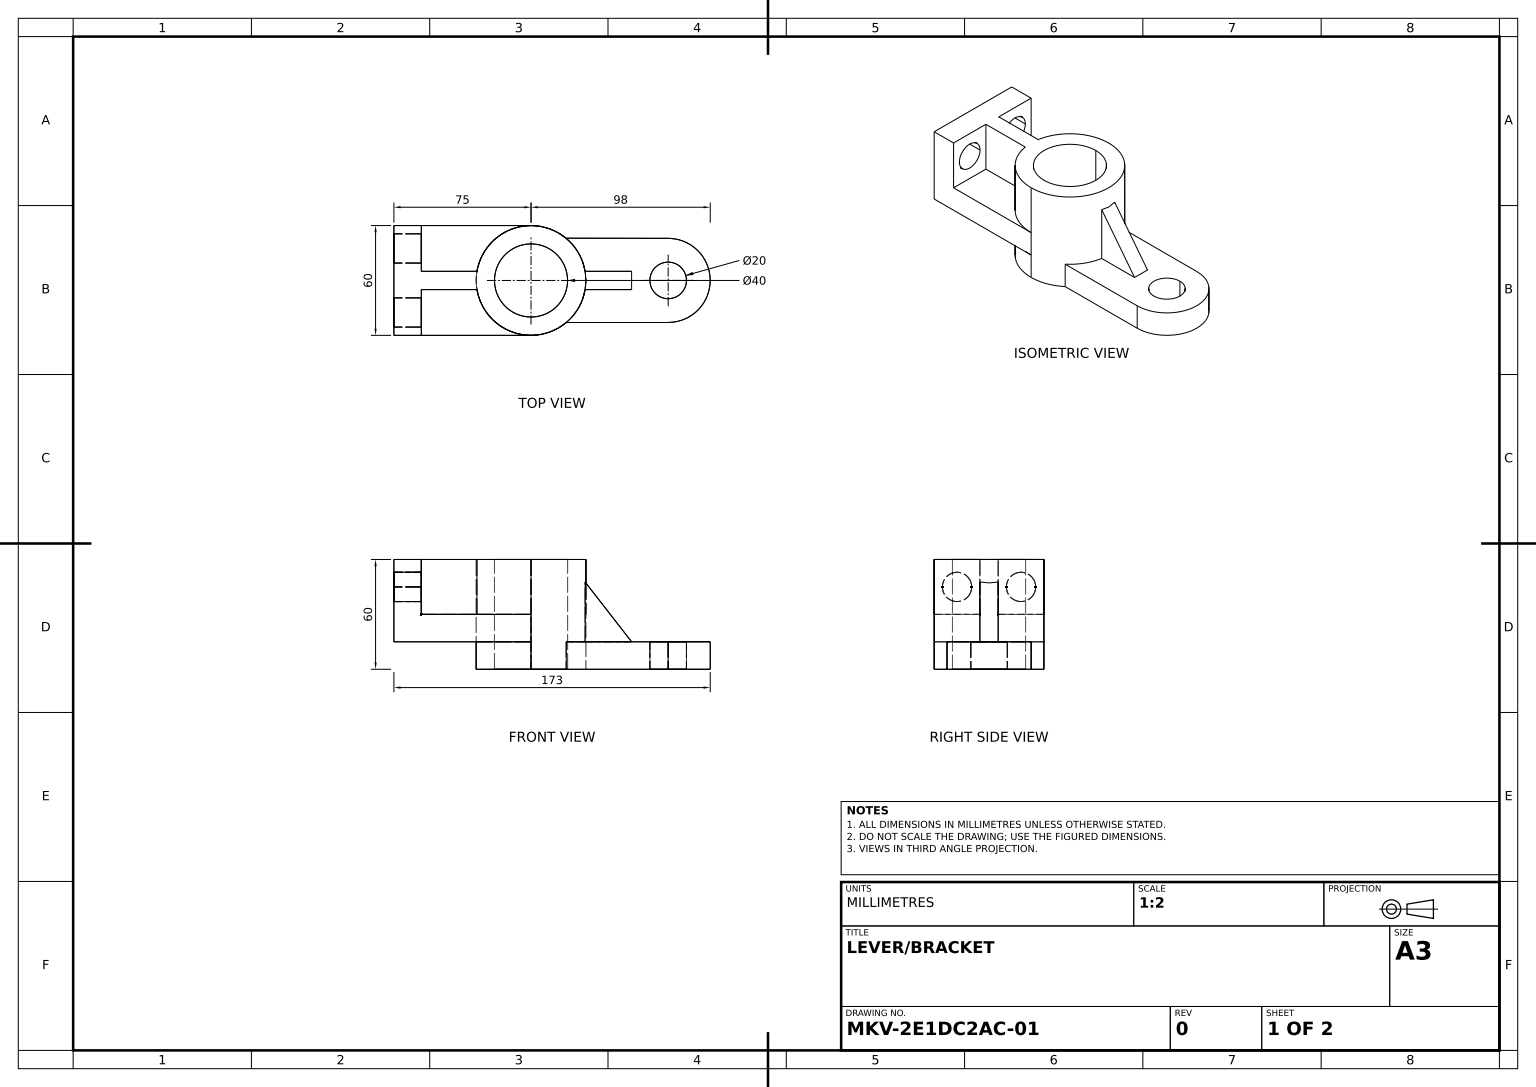
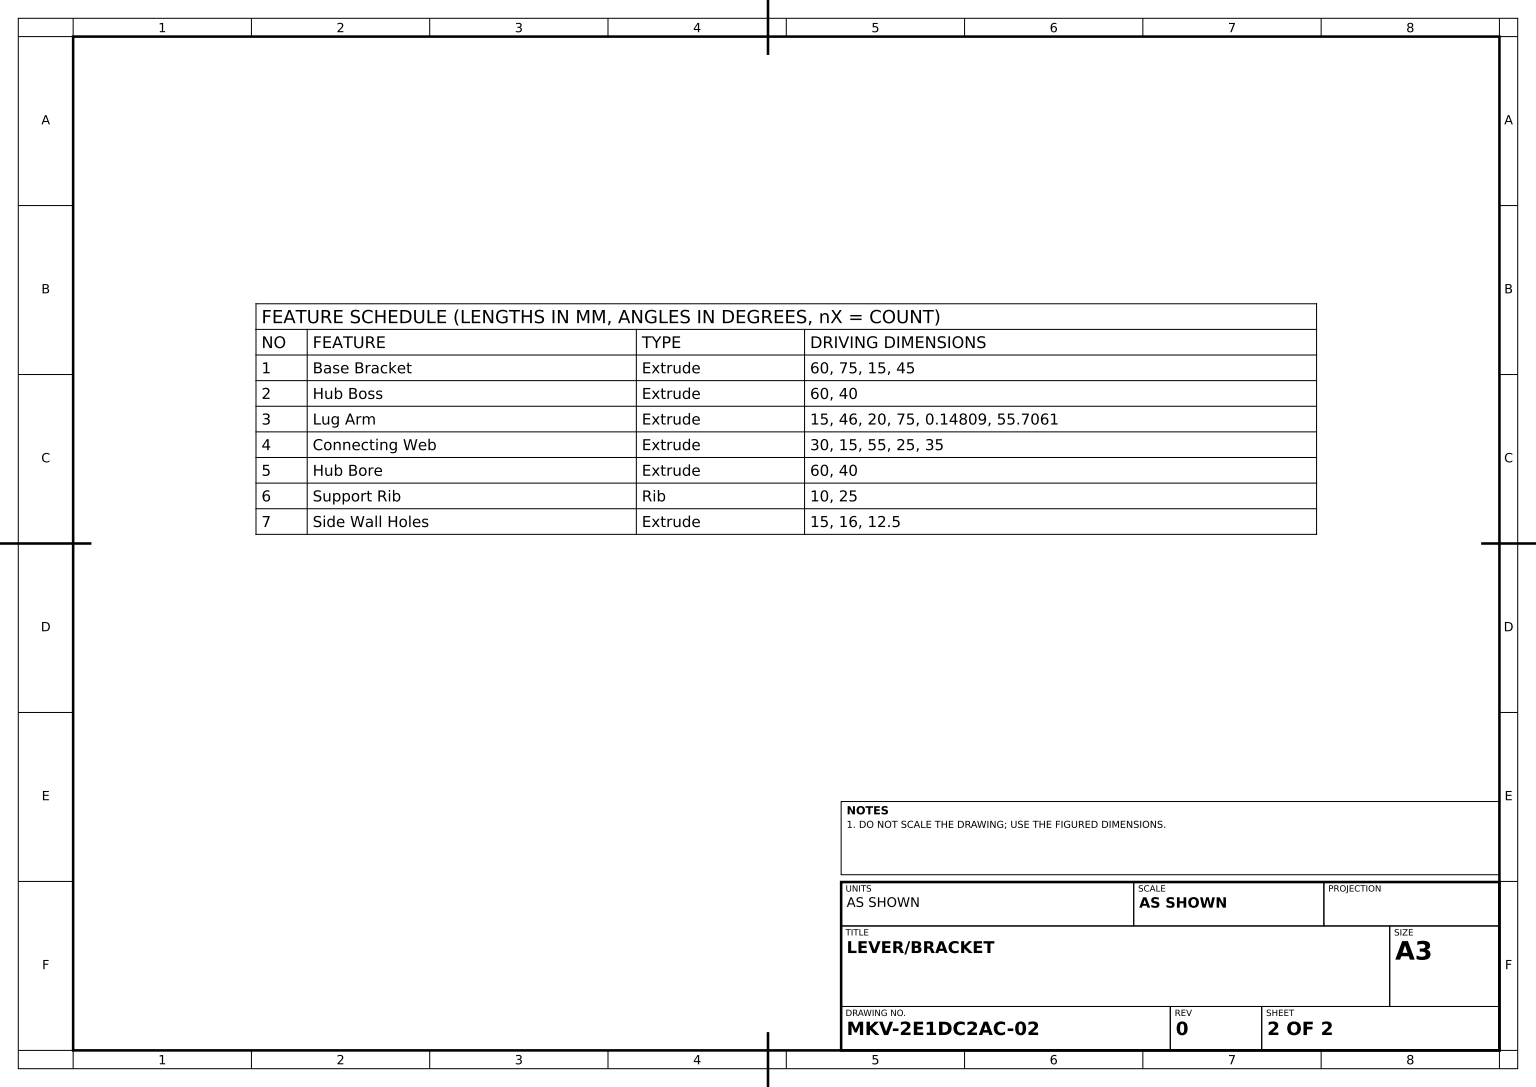
ISO-10303-21;
HEADER;
FILE_DESCRIPTION((''),'2;1');
FILE_NAME('','',(''),(''),'','','');
FILE_SCHEMA(('AUTOMOTIVE_DESIGN'));
ENDSEC;
DATA;
#1=APPLICATION_CONTEXT('');
#2=PRODUCT_CONTEXT('',#1,'mechanical');
#3=PRODUCT('','','',(#2));
#4=PRODUCT_DEFINITION_FORMATION('','',#3);
#5=PRODUCT_DEFINITION_CONTEXT('',#1,'design');
#6=PRODUCT_DEFINITION('','',#4,#5);
#7=PRODUCT_DEFINITION_SHAPE('','',#6);
#8=(LENGTH_UNIT()NAMED_UNIT(*)SI_UNIT(.MILLI.,.METRE.));
#9=(NAMED_UNIT(*)PLANE_ANGLE_UNIT()SI_UNIT($,.RADIAN.));
#10=(NAMED_UNIT(*)SI_UNIT($,.STERADIAN.)SOLID_ANGLE_UNIT());
#11=UNCERTAINTY_MEASURE_WITH_UNIT(LENGTH_MEASURE(1.E-05),#8,'distance_accuracy_value','');
#12=(GEOMETRIC_REPRESENTATION_CONTEXT(3)GLOBAL_UNCERTAINTY_ASSIGNED_CONTEXT((#11))GLOBAL_UNIT_ASSIGNED_CONTEXT((#8,#9,#10))REPRESENTATION_CONTEXT('',''));
#13=CARTESIAN_POINT('',(-60.,45.,9.5));
#14=VERTEX_POINT('',#13);
#15=CARTESIAN_POINT('',(-75.,45.,9.5));
#16=VERTEX_POINT('',#15);
#17=DIRECTION('',(-1.,0.,0.));
#18=VECTOR('',#17,1000.);
#19=LINE('',#13,#18);
#20=EDGE_CURVE('',#14,#16,#19,.T.);
#21=ORIENTED_EDGE('',*,*,#20,.F.);
#22=CARTESIAN_POINT('',(-60.,45.,25.5));
#23=VERTEX_POINT('',#22);
#24=CARTESIAN_POINT('',(-60.,45.,17.5));
#25=DIRECTION('',(0.,0.,1.));
#26=AXIS2_PLACEMENT_3D('',#24,#17,#25);
#27=CIRCLE('',#26,8.);
#28=EDGE_CURVE('',#23,#14,#27,.T.);
#29=ORIENTED_EDGE('',*,*,#28,.F.);
#30=CARTESIAN_POINT('',(-75.,45.,25.5));
#31=VERTEX_POINT('',#30);
#32=LINE('',#22,#18);
#33=EDGE_CURVE('',#23,#31,#32,.T.);
#34=ORIENTED_EDGE('',*,*,#33,.T.);
#35=CARTESIAN_POINT('',(-75.,45.,17.5));
#36=AXIS2_PLACEMENT_3D('',#35,#17,#25);
#37=CIRCLE('',#36,8.);
#38=EDGE_CURVE('',#31,#16,#37,.T.);
#39=ORIENTED_EDGE('',*,*,#38,.T.);
#40=EDGE_LOOP('',(#21,#29,#34,#39));
#41=FACE_OUTER_BOUND('',#40,.T.);
#42=CYLINDRICAL_SURFACE('',#26,8.);
#43=ADVANCED_FACE('',(#41),#42,.F.);
#44=CARTESIAN_POINT('',(-29.580399,60.,5.));
#45=VERTEX_POINT('',#44);
#46=CARTESIAN_POINT('',(-29.580399,30.,5.));
#47=VERTEX_POINT('',#46);
#48=DIRECTION('',(0.,-1.,0.));
#49=VECTOR('',#48,1000.);
#50=LINE('',#44,#49);
#51=EDGE_CURVE('',#45,#47,#50,.T.);
#52=ORIENTED_EDGE('',*,*,#51,.F.);
#53=CARTESIAN_POINT('',(-60.,60.,5.));
#54=VERTEX_POINT('',#53);
#55=DIRECTION('',(1.,0.,0.));
#56=VECTOR('',#55,1000.);
#57=LINE('',#53,#56);
#58=EDGE_CURVE('',#54,#45,#57,.T.);
#59=ORIENTED_EDGE('',*,*,#58,.F.);
#60=CARTESIAN_POINT('',(-60.,30.,5.));
#61=VERTEX_POINT('',#60);
#62=DIRECTION('',(0.,1.,0.));
#63=VECTOR('',#62,1000.);
#64=LINE('',#60,#63);
#65=EDGE_CURVE('',#61,#54,#64,.T.);
#66=ORIENTED_EDGE('',*,*,#65,.F.);
#67=LINE('',#60,#56);
#68=EDGE_CURVE('',#61,#47,#67,.T.);
#69=ORIENTED_EDGE('',*,*,#68,.T.);
#70=EDGE_LOOP('',(#52,#59,#66,#69));
#71=FACE_OUTER_BOUND('',#70,.T.);
#72=AXIS2_PLACEMENT_3D('',#60,#25,#55);
#73=PLANE('',#72);
#74=ADVANCED_FACE('',(#71),#73,.T.);
#75=CARTESIAN_POINT('',(29.580399,15.,5.));
#76=VERTEX_POINT('',#75);
#77=CARTESIAN_POINT('',(55.,15.,5.));
#78=VERTEX_POINT('',#77);
#79=CARTESIAN_POINT('',(74.999995,15.,5.));
#80=LINE('',#79,#56);
#81=EDGE_CURVE('',#76,#78,#80,.T.);
#82=ORIENTED_EDGE('',*,*,#81,.T.);
#83=CARTESIAN_POINT('',(29.580399,47.682344,5.));
#84=VERTEX_POINT('',#83);
#85=CARTESIAN_POINT('',(20.,60.,5.));
#86=DIRECTION('',(0.613940614,-0.789352217,0.));
#87=VECTOR('',#86,1000.);
#88=LINE('',#85,#87);
#89=EDGE_CURVE('',#84,#78,#88,.T.);
#90=ORIENTED_EDGE('',*,*,#89,.F.);
#91=CARTESIAN_POINT('',(29.580399,60.,5.));
#92=LINE('',#91,#63);
#93=EDGE_CURVE('',#76,#84,#92,.T.);
#94=ORIENTED_EDGE('',*,*,#93,.F.);
#95=EDGE_LOOP('',(#82,#90,#94));
#96=FACE_OUTER_BOUND('',#95,.T.);
#97=CARTESIAN_POINT('',(11.499998,30.,5.));
#98=AXIS2_PLACEMENT_3D('',#97,#25,#55);
#99=PLANE('',#98);
#100=ADVANCED_FACE('',(#96),#99,.T.);
#101=CARTESIAN_POINT('',(0.,60.,20.));
#102=VERTEX_POINT('',#101);
#103=CARTESIAN_POINT('',(0.,60.,-20.));
#104=VERTEX_POINT('',#103);
#105=CARTESIAN_POINT('',(0.,60.,0.));
#106=AXIS2_PLACEMENT_3D('',#105,#62,#25);
#107=CIRCLE('',#106,20.);
#108=EDGE_CURVE('',#102,#104,#107,.T.);
#109=ORIENTED_EDGE('',*,*,#108,.F.);
#110=EDGE_CURVE('',#104,#102,#107,.T.);
#111=ORIENTED_EDGE('',*,*,#110,.F.);
#112=EDGE_LOOP('',(#109,#111));
#113=FACE_BOUND('',#112,.T.);
#114=CARTESIAN_POINT('',(0.,60.,30.));
#115=VERTEX_POINT('',#114);
#116=CARTESIAN_POINT('',(0.,60.,-30.));
#117=VERTEX_POINT('',#116);
#118=CIRCLE('',#106,30.);
#119=EDGE_CURVE('',#115,#117,#118,.T.);
#120=ORIENTED_EDGE('',*,*,#119,.T.);
#121=CARTESIAN_POINT('',(-29.580399,60.,-5.));
#122=VERTEX_POINT('',#121);
#123=EDGE_CURVE('',#117,#122,#118,.T.);
#124=ORIENTED_EDGE('',*,*,#123,.T.);
#125=CARTESIAN_POINT('',(-60.,60.,-5.));
#126=VERTEX_POINT('',#125);
#127=LINE('',#125,#18);
#128=EDGE_CURVE('',#122,#126,#127,.T.);
#129=ORIENTED_EDGE('',*,*,#128,.T.);
#130=CARTESIAN_POINT('',(-60.,60.,-30.));
#131=VERTEX_POINT('',#130);
#132=CARTESIAN_POINT('',(-60.,60.,30.));
#133=DIRECTION('',(0.,0.,-1.));
#134=VECTOR('',#133,1000.);
#135=LINE('',#132,#134);
#136=EDGE_CURVE('',#126,#131,#135,.T.);
#137=ORIENTED_EDGE('',*,*,#136,.T.);
#138=CARTESIAN_POINT('',(-75.,60.,-30.));
#139=VERTEX_POINT('',#138);
#140=LINE('',#138,#18);
#141=EDGE_CURVE('',#131,#139,#140,.T.);
#142=ORIENTED_EDGE('',*,*,#141,.T.);
#143=CARTESIAN_POINT('',(-75.,60.,30.));
#144=VERTEX_POINT('',#143);
#145=LINE('',#143,#134);
#146=EDGE_CURVE('',#144,#139,#145,.T.);
#147=ORIENTED_EDGE('',*,*,#146,.F.);
#148=VERTEX_POINT('',#132);
#149=LINE('',#143,#18);
#150=EDGE_CURVE('',#148,#144,#149,.T.);
#151=ORIENTED_EDGE('',*,*,#150,.F.);
#152=EDGE_CURVE('',#148,#54,#135,.T.);
#153=ORIENTED_EDGE('',*,*,#152,.T.);
#154=ORIENTED_EDGE('',*,*,#58,.T.);
#155=EDGE_CURVE('',#45,#115,#118,.T.);
#156=ORIENTED_EDGE('',*,*,#155,.T.);
#157=EDGE_LOOP('',(#120,#124,#129,#137,#142,#147,#151,#153,#154,#156));
#158=FACE_OUTER_BOUND('',#157,.T.);
#159=AXIS2_PLACEMENT_3D('',#143,#48,#55);
#160=PLANE('',#159);
#161=ADVANCED_FACE('',(#113,#158),#160,.F.);
#162=ORIENTED_EDGE('',*,*,#20,.T.);
#163=EDGE_CURVE('',#16,#31,#37,.T.);
#164=ORIENTED_EDGE('',*,*,#163,.T.);
#165=ORIENTED_EDGE('',*,*,#33,.F.);
#166=EDGE_CURVE('',#14,#23,#27,.T.);
#167=ORIENTED_EDGE('',*,*,#166,.F.);
#168=EDGE_LOOP('',(#162,#164,#165,#167));
#169=FACE_OUTER_BOUND('',#168,.T.);
#170=ADVANCED_FACE('',(#169),#42,.F.);
#171=CARTESIAN_POINT('',(-60.,45.,-25.5));
#172=VERTEX_POINT('',#171);
#173=CARTESIAN_POINT('',(-60.,45.,-9.5));
#174=VERTEX_POINT('',#173);
#175=CARTESIAN_POINT('',(-60.,45.,-17.5));
#176=AXIS2_PLACEMENT_3D('',#175,#17,#25);
#177=CIRCLE('',#176,8.);
#178=EDGE_CURVE('',#172,#174,#177,.T.);
#179=ORIENTED_EDGE('',*,*,#178,.T.);
#180=EDGE_CURVE('',#174,#172,#177,.T.);
#181=ORIENTED_EDGE('',*,*,#180,.T.);
#182=EDGE_LOOP('',(#179,#181));
#183=FACE_BOUND('',#182,.T.);
#184=CARTESIAN_POINT('',(-60.,30.,-5.));
#185=VERTEX_POINT('',#184);
#186=LINE('',#184,#63);
#187=EDGE_CURVE('',#185,#126,#186,.T.);
#188=ORIENTED_EDGE('',*,*,#187,.F.);
#189=CARTESIAN_POINT('',(-60.,30.,-30.));
#190=VERTEX_POINT('',#189);
#191=CARTESIAN_POINT('',(-60.,30.,30.));
#192=LINE('',#191,#134);
#193=EDGE_CURVE('',#185,#190,#192,.T.);
#194=ORIENTED_EDGE('',*,*,#193,.T.);
#195=LINE('',#130,#63);
#196=EDGE_CURVE('',#190,#131,#195,.T.);
#197=ORIENTED_EDGE('',*,*,#196,.T.);
#198=ORIENTED_EDGE('',*,*,#136,.F.);
#199=EDGE_LOOP('',(#188,#194,#197,#198));
#200=FACE_OUTER_BOUND('',#199,.T.);
#201=AXIS2_PLACEMENT_3D('',#132,#17,#48);
#202=PLANE('',#201);
#203=ADVANCED_FACE('',(#183,#200),#202,.F.);
#204=CARTESIAN_POINT('',(-75.,15.,30.));
#205=VERTEX_POINT('',#204);
#206=CARTESIAN_POINT('',(0.,15.,30.));
#207=VERTEX_POINT('',#206);
#208=LINE('',#206,#56);
#209=EDGE_CURVE('',#205,#207,#208,.T.);
#210=ORIENTED_EDGE('',*,*,#209,.T.);
#211=CARTESIAN_POINT('',(0.,30.,30.));
#212=VERTEX_POINT('',#211);
#213=LINE('',#211,#63);
#214=EDGE_CURVE('',#207,#212,#213,.T.);
#215=ORIENTED_EDGE('',*,*,#214,.T.);
#216=VERTEX_POINT('',#191);
#217=LINE('',#191,#18);
#218=EDGE_CURVE('',#212,#216,#217,.T.);
#219=ORIENTED_EDGE('',*,*,#218,.T.);
#220=LINE('',#132,#63);
#221=EDGE_CURVE('',#216,#148,#220,.T.);
#222=ORIENTED_EDGE('',*,*,#221,.T.);
#223=ORIENTED_EDGE('',*,*,#150,.T.);
#224=LINE('',#204,#49);
#225=EDGE_CURVE('',#144,#205,#224,.T.);
#226=ORIENTED_EDGE('',*,*,#225,.T.);
#227=EDGE_LOOP('',(#210,#215,#219,#222,#223,#226));
#228=FACE_OUTER_BOUND('',#227,.T.);
#229=CARTESIAN_POINT('',(0.,0.,30.));
#230=AXIS2_PLACEMENT_3D('',#229,#133,#17);
#231=PLANE('',#230);
#232=ADVANCED_FACE('',(#228),#231,.F.);
#233=CARTESIAN_POINT('',(0.,0.,20.));
#234=VERTEX_POINT('',#233);
#235=CARTESIAN_POINT('',(0.,0.,-20.));
#236=VERTEX_POINT('',#235);
#237=CARTESIAN_POINT('',(0.,0.,0.));
#238=AXIS2_PLACEMENT_3D('',#237,#62,#25);
#239=CIRCLE('',#238,20.);
#240=EDGE_CURVE('',#234,#236,#239,.T.);
#241=ORIENTED_EDGE('',*,*,#240,.T.);
#242=EDGE_CURVE('',#236,#234,#239,.T.);
#243=ORIENTED_EDGE('',*,*,#242,.T.);
#244=EDGE_LOOP('',(#241,#243));
#245=FACE_BOUND('',#244,.T.);
#246=VERTEX_POINT('',#229);
#247=CARTESIAN_POINT('',(19.293898,0.,22.972712));
#248=VERTEX_POINT('',#247);
#249=CIRCLE('',#238,30.);
#250=EDGE_CURVE('',#246,#248,#249,.T.);
#251=ORIENTED_EDGE('',*,*,#250,.F.);
#252=CARTESIAN_POINT('',(0.,0.,-30.));
#253=VERTEX_POINT('',#252);
#254=EDGE_CURVE('',#253,#246,#249,.T.);
#255=ORIENTED_EDGE('',*,*,#254,.F.);
#256=CARTESIAN_POINT('',(19.145809,0.,-23.096277));
#257=VERTEX_POINT('',#256);
#258=EDGE_CURVE('',#257,#253,#249,.T.);
#259=ORIENTED_EDGE('',*,*,#258,.F.);
#260=CARTESIAN_POINT('',(74.999995,0.,-23.027288));
#261=VERTEX_POINT('',#260);
#262=DIRECTION('',(-0.999999237,0.,-0.001235159));
#263=VECTOR('',#262,1000.);
#264=LINE('',#260,#263);
#265=EDGE_CURVE('',#261,#257,#264,.T.);
#266=ORIENTED_EDGE('',*,*,#265,.F.);
#267=CARTESIAN_POINT('',(74.999995,0.,22.972712));
#268=VERTEX_POINT('',#267);
#269=CARTESIAN_POINT('',(74.999995,0.,-0.027288));
#270=AXIS2_PLACEMENT_3D('',#269,#62,#25);
#271=CIRCLE('',#270,23.);
#272=EDGE_CURVE('',#268,#261,#271,.T.);
#273=ORIENTED_EDGE('',*,*,#272,.F.);
#274=LINE('',#247,#56);
#275=EDGE_CURVE('',#248,#268,#274,.T.);
#276=ORIENTED_EDGE('',*,*,#275,.F.);
#277=EDGE_LOOP('',(#251,#255,#259,#266,#273,#276));
#278=FACE_OUTER_BOUND('',#277,.T.);
#279=CARTESIAN_POINT('',(74.999995,0.,-10.027288));
#280=VERTEX_POINT('',#279);
#281=CARTESIAN_POINT('',(74.999995,0.,9.972712));
#282=VERTEX_POINT('',#281);
#283=CIRCLE('',#270,10.);
#284=EDGE_CURVE('',#280,#282,#283,.T.);
#285=ORIENTED_EDGE('',*,*,#284,.T.);
#286=EDGE_CURVE('',#282,#280,#283,.T.);
#287=ORIENTED_EDGE('',*,*,#286,.T.);
#288=EDGE_LOOP('',(#285,#287));
#289=FACE_BOUND('',#288,.T.);
#290=PLANE('',#238);
#291=ADVANCED_FACE('',(#245,#278,#289),#290,.F.);
#292=CARTESIAN_POINT('',(29.580399,47.682344,-5.));
#293=VERTEX_POINT('',#292);
#294=CARTESIAN_POINT('',(55.,15.,-5.));
#295=VERTEX_POINT('',#294);
#296=CARTESIAN_POINT('',(20.,60.,-5.));
#297=LINE('',#296,#87);
#298=EDGE_CURVE('',#293,#295,#297,.T.);
#299=ORIENTED_EDGE('',*,*,#298,.F.);
#300=CARTESIAN_POINT('',(30.141183,46.961336,1.682354));
#301=CARTESIAN_POINT('',(30.141183,46.961336,-1.682354));
#302=(BOUNDED_CURVE()B_SPLINE_CURVE(3,(#83,#300,#301,#292),.UNSPECIFIED.,.F.,.F.)B_SPLINE_CURVE_WITH_KNOTS((4,4),(6.115737228,6.450633386),.UNSPECIFIED.)CURVE()GEOMETRIC_REPRESENTATION_ITEM()RATIONAL_B_SPLINE_CURVE((1.,0.990675531,0.990675531,1.))REPRESENTATION_ITEM(''));
#303=EDGE_CURVE('',#84,#293,#302,.T.);
#304=ORIENTED_EDGE('',*,*,#303,.F.);
#305=ORIENTED_EDGE('',*,*,#89,.T.);
#306=CARTESIAN_POINT('',(55.,15.,-0.027288));
#307=LINE('',#306,#134);
#308=EDGE_CURVE('',#78,#295,#307,.T.);
#309=ORIENTED_EDGE('',*,*,#308,.T.);
#310=EDGE_LOOP('',(#299,#304,#305,#309));
#311=FACE_OUTER_BOUND('',#310,.T.);
#312=CARTESIAN_POINT('',(20.,60.,0.));
#313=DIRECTION('',(-0.789352217,-0.613940614,0.));
#314=AXIS2_PLACEMENT_3D('',#312,#313,#86);
#315=PLANE('',#314);
#316=ADVANCED_FACE('',(#311),#315,.F.);
#317=CARTESIAN_POINT('',(-75.,45.,-25.5));
#318=VERTEX_POINT('',#317);
#319=LINE('',#171,#18);
#320=EDGE_CURVE('',#172,#318,#319,.T.);
#321=ORIENTED_EDGE('',*,*,#320,.T.);
#322=CARTESIAN_POINT('',(-75.,45.,-9.5));
#323=VERTEX_POINT('',#322);
#324=CARTESIAN_POINT('',(-75.,45.,-17.5));
#325=AXIS2_PLACEMENT_3D('',#324,#17,#25);
#326=CIRCLE('',#325,8.);
#327=EDGE_CURVE('',#318,#323,#326,.T.);
#328=ORIENTED_EDGE('',*,*,#327,.T.);
#329=LINE('',#173,#18);
#330=EDGE_CURVE('',#174,#323,#329,.T.);
#331=ORIENTED_EDGE('',*,*,#330,.F.);
#332=ORIENTED_EDGE('',*,*,#178,.F.);
#333=EDGE_LOOP('',(#321,#328,#331,#332));
#334=FACE_OUTER_BOUND('',#333,.T.);
#335=CYLINDRICAL_SURFACE('',#176,8.);
#336=ADVANCED_FACE('',(#334),#335,.F.);
#337=ORIENTED_EDGE('',*,*,#214,.F.);
#338=LINE('',#114,#49);
#339=EDGE_CURVE('',#207,#246,#338,.T.);
#340=ORIENTED_EDGE('',*,*,#339,.T.);
#341=ORIENTED_EDGE('',*,*,#250,.T.);
#342=CARTESIAN_POINT('',(19.293898,15.,22.972712));
#343=VERTEX_POINT('',#342);
#344=LINE('',#342,#49);
#345=EDGE_CURVE('',#343,#248,#344,.T.);
#346=ORIENTED_EDGE('',*,*,#345,.F.);
#347=CARTESIAN_POINT('',(0.,15.,0.));
#348=AXIS2_PLACEMENT_3D('',#347,#62,#25);
#349=CIRCLE('',#348,30.);
#350=EDGE_CURVE('',#343,#76,#349,.T.);
#351=ORIENTED_EDGE('',*,*,#350,.T.);
#352=ORIENTED_EDGE('',*,*,#93,.T.);
#353=ORIENTED_EDGE('',*,*,#303,.T.);
#354=CARTESIAN_POINT('',(29.580399,15.,-5.));
#355=VERTEX_POINT('',#354);
#356=CARTESIAN_POINT('',(29.580399,60.,-5.));
#357=LINE('',#356,#63);
#358=EDGE_CURVE('',#355,#293,#357,.T.);
#359=ORIENTED_EDGE('',*,*,#358,.F.);
#360=CARTESIAN_POINT('',(19.145809,15.,-23.096277));
#361=VERTEX_POINT('',#360);
#362=EDGE_CURVE('',#355,#361,#349,.T.);
#363=ORIENTED_EDGE('',*,*,#362,.T.);
#364=LINE('',#360,#49);
#365=EDGE_CURVE('',#361,#257,#364,.T.);
#366=ORIENTED_EDGE('',*,*,#365,.T.);
#367=ORIENTED_EDGE('',*,*,#258,.T.);
#368=CARTESIAN_POINT('',(0.,15.,-30.));
#369=VERTEX_POINT('',#368);
#370=LINE('',#116,#49);
#371=EDGE_CURVE('',#369,#253,#370,.T.);
#372=ORIENTED_EDGE('',*,*,#371,.F.);
#373=CARTESIAN_POINT('',(0.,30.,-30.));
#374=VERTEX_POINT('',#373);
#375=LINE('',#373,#63);
#376=EDGE_CURVE('',#369,#374,#375,.T.);
#377=ORIENTED_EDGE('',*,*,#376,.T.);
#378=EDGE_CURVE('',#117,#374,#370,.T.);
#379=ORIENTED_EDGE('',*,*,#378,.F.);
#380=ORIENTED_EDGE('',*,*,#119,.F.);
#381=EDGE_CURVE('',#115,#212,#338,.T.);
#382=ORIENTED_EDGE('',*,*,#381,.T.);
#383=EDGE_LOOP('',(#337,#340,#341,#346,#351,#352,#353,#359,#363,#366,#367,#372,#377,#379,#380,#382));
#384=FACE_OUTER_BOUND('',#383,.T.);
#385=AXIS2_PLACEMENT_3D('',#105,#48,#133);
#386=CYLINDRICAL_SURFACE('',#385,30.);
#387=ADVANCED_FACE('',(#384),#386,.T.);
#388=ORIENTED_EDGE('',*,*,#108,.T.);
#389=LINE('',#103,#49);
#390=EDGE_CURVE('',#104,#236,#389,.T.);
#391=ORIENTED_EDGE('',*,*,#390,.T.);
#392=ORIENTED_EDGE('',*,*,#240,.F.);
#393=LINE('',#101,#49);
#394=EDGE_CURVE('',#102,#234,#393,.T.);
#395=ORIENTED_EDGE('',*,*,#394,.F.);
#396=EDGE_LOOP('',(#388,#391,#392,#395));
#397=FACE_OUTER_BOUND('',#396,.T.);
#398=CYLINDRICAL_SURFACE('',#385,20.);
#399=ADVANCED_FACE('',(#397),#398,.F.);
#400=CARTESIAN_POINT('',(-75.,15.,-30.));
#401=VERTEX_POINT('',#400);
#402=LINE('',#368,#56);
#403=EDGE_CURVE('',#401,#369,#402,.T.);
#404=ORIENTED_EDGE('',*,*,#403,.F.);
#405=LINE('',#400,#49);
#406=EDGE_CURVE('',#139,#401,#405,.T.);
#407=ORIENTED_EDGE('',*,*,#406,.F.);
#408=ORIENTED_EDGE('',*,*,#141,.F.);
#409=ORIENTED_EDGE('',*,*,#196,.F.);
#410=LINE('',#189,#18);
#411=EDGE_CURVE('',#374,#190,#410,.T.);
#412=ORIENTED_EDGE('',*,*,#411,.F.);
#413=ORIENTED_EDGE('',*,*,#376,.F.);
#414=EDGE_LOOP('',(#404,#407,#408,#409,#412,#413));
#415=FACE_OUTER_BOUND('',#414,.T.);
#416=AXIS2_PLACEMENT_3D('',#252,#133,#17);
#417=PLANE('',#416);
#418=ADVANCED_FACE('',(#415),#417,.T.);
#419=CARTESIAN_POINT('',(74.999995,15.,22.972712));
#420=VERTEX_POINT('',#419);
#421=LINE('',#419,#49);
#422=EDGE_CURVE('',#420,#268,#421,.T.);
#423=ORIENTED_EDGE('',*,*,#422,.F.);
#424=LINE('',#342,#56);
#425=EDGE_CURVE('',#343,#420,#424,.T.);
#426=ORIENTED_EDGE('',*,*,#425,.F.);
#427=ORIENTED_EDGE('',*,*,#345,.T.);
#428=ORIENTED_EDGE('',*,*,#275,.T.);
#429=EDGE_LOOP('',(#423,#426,#427,#428));
#430=FACE_OUTER_BOUND('',#429,.T.);
#431=AXIS2_PLACEMENT_3D('',#342,#133,#17);
#432=PLANE('',#431);
#433=ADVANCED_FACE('',(#430),#432,.F.);
#434=ORIENTED_EDGE('',*,*,#218,.F.);
#435=CARTESIAN_POINT('',(0.,30.,0.));
#436=AXIS2_PLACEMENT_3D('',#435,#62,#133);
#437=CIRCLE('',#436,30.);
#438=EDGE_CURVE('',#47,#212,#437,.T.);
#439=ORIENTED_EDGE('',*,*,#438,.F.);
#440=ORIENTED_EDGE('',*,*,#68,.F.);
#441=EDGE_CURVE('',#216,#61,#192,.T.);
#442=ORIENTED_EDGE('',*,*,#441,.F.);
#443=EDGE_LOOP('',(#434,#439,#440,#442));
#444=FACE_OUTER_BOUND('',#443,.T.);
#445=AXIS2_PLACEMENT_3D('',#191,#48,#133);
#446=PLANE('',#445);
#447=ADVANCED_FACE('',(#444),#446,.F.);
#448=CARTESIAN_POINT('',(74.999995,15.,-23.027288));
#449=VERTEX_POINT('',#448);
#450=CARTESIAN_POINT('',(74.999995,15.,-0.027288));
#451=AXIS2_PLACEMENT_3D('',#450,#62,#25);
#452=CIRCLE('',#451,23.);
#453=EDGE_CURVE('',#420,#449,#452,.T.);
#454=ORIENTED_EDGE('',*,*,#453,.T.);
#455=LINE('',#448,#263);
#456=EDGE_CURVE('',#449,#361,#455,.T.);
#457=ORIENTED_EDGE('',*,*,#456,.T.);
#458=ORIENTED_EDGE('',*,*,#362,.F.);
#459=CARTESIAN_POINT('',(74.999995,15.,-5.));
#460=LINE('',#459,#56);
#461=EDGE_CURVE('',#355,#295,#460,.T.);
#462=ORIENTED_EDGE('',*,*,#461,.T.);
#463=ORIENTED_EDGE('',*,*,#308,.F.);
#464=ORIENTED_EDGE('',*,*,#81,.F.);
#465=ORIENTED_EDGE('',*,*,#350,.F.);
#466=ORIENTED_EDGE('',*,*,#425,.T.);
#467=EDGE_LOOP('',(#454,#457,#458,#462,#463,#464,#465,#466));
#468=FACE_OUTER_BOUND('',#467,.T.);
#469=CARTESIAN_POINT('',(74.999995,15.,9.972712));
#470=VERTEX_POINT('',#469);
#471=CARTESIAN_POINT('',(74.999995,15.,-10.027288));
#472=VERTEX_POINT('',#471);
#473=CIRCLE('',#451,10.);
#474=EDGE_CURVE('',#470,#472,#473,.T.);
#475=ORIENTED_EDGE('',*,*,#474,.F.);
#476=EDGE_CURVE('',#472,#470,#473,.T.);
#477=ORIENTED_EDGE('',*,*,#476,.F.);
#478=EDGE_LOOP('',(#475,#477));
#479=FACE_BOUND('',#478,.T.);
#480=PLANE('',#451);
#481=ADVANCED_FACE('',(#468,#479),#480,.T.);
#482=ORIENTED_EDGE('',*,*,#453,.F.);
#483=ORIENTED_EDGE('',*,*,#422,.T.);
#484=ORIENTED_EDGE('',*,*,#272,.T.);
#485=LINE('',#448,#49);
#486=EDGE_CURVE('',#449,#261,#485,.T.);
#487=ORIENTED_EDGE('',*,*,#486,.F.);
#488=EDGE_LOOP('',(#482,#483,#484,#487));
#489=FACE_OUTER_BOUND('',#488,.T.);
#490=AXIS2_PLACEMENT_3D('',#450,#48,#133);
#491=CYLINDRICAL_SURFACE('',#490,23.);
#492=ADVANCED_FACE('',(#489),#491,.T.);
#493=ORIENTED_EDGE('',*,*,#298,.T.);
#494=ORIENTED_EDGE('',*,*,#461,.F.);
#495=ORIENTED_EDGE('',*,*,#358,.T.);
#496=EDGE_LOOP('',(#493,#494,#495));
#497=FACE_OUTER_BOUND('',#496,.T.);
#498=CARTESIAN_POINT('',(11.499998,30.,-5.));
#499=AXIS2_PLACEMENT_3D('',#498,#25,#55);
#500=PLANE('',#499);
#501=ADVANCED_FACE('',(#497),#500,.F.);
#502=ORIENTED_EDGE('',*,*,#152,.F.);
#503=ORIENTED_EDGE('',*,*,#221,.F.);
#504=ORIENTED_EDGE('',*,*,#441,.T.);
#505=ORIENTED_EDGE('',*,*,#65,.T.);
#506=EDGE_LOOP('',(#502,#503,#504,#505));
#507=FACE_OUTER_BOUND('',#506,.T.);
#508=ORIENTED_EDGE('',*,*,#166,.T.);
#509=ORIENTED_EDGE('',*,*,#28,.T.);
#510=EDGE_LOOP('',(#508,#509));
#511=FACE_BOUND('',#510,.T.);
#512=ADVANCED_FACE('',(#507,#511),#202,.F.);
#513=ORIENTED_EDGE('',*,*,#403,.T.);
#514=AXIS2_PLACEMENT_3D('',#347,#48,#17);
#515=CIRCLE('',#514,30.);
#516=EDGE_CURVE('',#207,#369,#515,.T.);
#517=ORIENTED_EDGE('',*,*,#516,.F.);
#518=ORIENTED_EDGE('',*,*,#209,.F.);
#519=LINE('',#204,#134);
#520=EDGE_CURVE('',#205,#401,#519,.T.);
#521=ORIENTED_EDGE('',*,*,#520,.T.);
#522=EDGE_LOOP('',(#513,#517,#518,#521));
#523=FACE_OUTER_BOUND('',#522,.T.);
#524=AXIS2_PLACEMENT_3D('',#206,#62,#17);
#525=PLANE('',#524);
#526=ADVANCED_FACE('',(#523),#525,.F.);
#527=CARTESIAN_POINT('',(-29.580399,30.,-5.));
#528=VERTEX_POINT('',#527);
#529=EDGE_CURVE('',#374,#528,#437,.T.);
#530=ORIENTED_EDGE('',*,*,#529,.F.);
#531=ORIENTED_EDGE('',*,*,#411,.T.);
#532=ORIENTED_EDGE('',*,*,#193,.F.);
#533=LINE('',#184,#18);
#534=EDGE_CURVE('',#528,#185,#533,.T.);
#535=ORIENTED_EDGE('',*,*,#534,.F.);
#536=EDGE_LOOP('',(#530,#531,#532,#535));
#537=FACE_OUTER_BOUND('',#536,.T.);
#538=ADVANCED_FACE('',(#537),#446,.F.);
#539=ORIENTED_EDGE('',*,*,#516,.T.);
#540=ORIENTED_EDGE('',*,*,#371,.T.);
#541=ORIENTED_EDGE('',*,*,#254,.T.);
#542=ORIENTED_EDGE('',*,*,#339,.F.);
#543=EDGE_LOOP('',(#539,#540,#541,#542));
#544=FACE_OUTER_BOUND('',#543,.T.);
#545=ADVANCED_FACE('',(#544),#386,.T.);
#546=ORIENTED_EDGE('',*,*,#474,.T.);
#547=LINE('',#471,#49);
#548=EDGE_CURVE('',#472,#280,#547,.T.);
#549=ORIENTED_EDGE('',*,*,#548,.T.);
#550=ORIENTED_EDGE('',*,*,#286,.F.);
#551=LINE('',#469,#49);
#552=EDGE_CURVE('',#470,#282,#551,.T.);
#553=ORIENTED_EDGE('',*,*,#552,.F.);
#554=EDGE_LOOP('',(#546,#549,#550,#553));
#555=FACE_OUTER_BOUND('',#554,.T.);
#556=CYLINDRICAL_SURFACE('',#490,10.);
#557=ADVANCED_FACE('',(#555),#556,.F.);
#558=EDGE_CURVE('',#323,#318,#326,.T.);
#559=ORIENTED_EDGE('',*,*,#558,.T.);
#560=ORIENTED_EDGE('',*,*,#320,.F.);
#561=ORIENTED_EDGE('',*,*,#180,.F.);
#562=ORIENTED_EDGE('',*,*,#330,.T.);
#563=EDGE_LOOP('',(#559,#560,#561,#562));
#564=FACE_OUTER_BOUND('',#563,.T.);
#565=ADVANCED_FACE('',(#564),#335,.F.);
#566=ORIENTED_EDGE('',*,*,#284,.F.);
#567=ORIENTED_EDGE('',*,*,#548,.F.);
#568=ORIENTED_EDGE('',*,*,#476,.T.);
#569=ORIENTED_EDGE('',*,*,#552,.T.);
#570=EDGE_LOOP('',(#566,#567,#568,#569));
#571=FACE_OUTER_BOUND('',#570,.T.);
#572=ADVANCED_FACE('',(#571),#556,.F.);
#573=ORIENTED_EDGE('',*,*,#327,.F.);
#574=ORIENTED_EDGE('',*,*,#558,.F.);
#575=EDGE_LOOP('',(#573,#574));
#576=FACE_BOUND('',#575,.T.);
#577=ORIENTED_EDGE('',*,*,#520,.F.);
#578=ORIENTED_EDGE('',*,*,#225,.F.);
#579=ORIENTED_EDGE('',*,*,#146,.T.);
#580=ORIENTED_EDGE('',*,*,#406,.T.);
#581=EDGE_LOOP('',(#577,#578,#579,#580));
#582=FACE_OUTER_BOUND('',#581,.T.);
#583=ORIENTED_EDGE('',*,*,#38,.F.);
#584=ORIENTED_EDGE('',*,*,#163,.F.);
#585=EDGE_LOOP('',(#583,#584));
#586=FACE_BOUND('',#585,.T.);
#587=AXIS2_PLACEMENT_3D('',#204,#55,#133);
#588=PLANE('',#587);
#589=ADVANCED_FACE('',(#576,#582,#586),#588,.F.);
#590=ORIENTED_EDGE('',*,*,#456,.F.);
#591=ORIENTED_EDGE('',*,*,#486,.T.);
#592=ORIENTED_EDGE('',*,*,#265,.T.);
#593=ORIENTED_EDGE('',*,*,#365,.F.);
#594=EDGE_LOOP('',(#590,#591,#592,#593));
#595=FACE_OUTER_BOUND('',#594,.T.);
#596=DIRECTION('',(-0.001235159,0.,0.999999237));
#597=DIRECTION('',(0.999999237,0.,0.001235159));
#598=AXIS2_PLACEMENT_3D('',#448,#596,#597);
#599=PLANE('',#598);
#600=ADVANCED_FACE('',(#595),#599,.F.);
#601=ORIENTED_EDGE('',*,*,#529,.T.);
#602=LINE('',#121,#63);
#603=EDGE_CURVE('',#528,#122,#602,.T.);
#604=ORIENTED_EDGE('',*,*,#603,.T.);
#605=ORIENTED_EDGE('',*,*,#123,.F.);
#606=ORIENTED_EDGE('',*,*,#378,.T.);
#607=EDGE_LOOP('',(#601,#604,#605,#606));
#608=FACE_OUTER_BOUND('',#607,.T.);
#609=ADVANCED_FACE('',(#608),#386,.T.);
#610=ORIENTED_EDGE('',*,*,#155,.F.);
#611=ORIENTED_EDGE('',*,*,#51,.T.);
#612=ORIENTED_EDGE('',*,*,#438,.T.);
#613=ORIENTED_EDGE('',*,*,#381,.F.);
#614=EDGE_LOOP('',(#610,#611,#612,#613));
#615=FACE_OUTER_BOUND('',#614,.T.);
#616=ADVANCED_FACE('',(#615),#386,.T.);
#617=ORIENTED_EDGE('',*,*,#242,.F.);
#618=ORIENTED_EDGE('',*,*,#390,.F.);
#619=ORIENTED_EDGE('',*,*,#110,.T.);
#620=ORIENTED_EDGE('',*,*,#394,.T.);
#621=EDGE_LOOP('',(#617,#618,#619,#620));
#622=FACE_OUTER_BOUND('',#621,.T.);
#623=ADVANCED_FACE('',(#622),#398,.F.);
#624=ORIENTED_EDGE('',*,*,#534,.T.);
#625=ORIENTED_EDGE('',*,*,#187,.T.);
#626=ORIENTED_EDGE('',*,*,#128,.F.);
#627=ORIENTED_EDGE('',*,*,#603,.F.);
#628=EDGE_LOOP('',(#624,#625,#626,#627));
#629=FACE_OUTER_BOUND('',#628,.T.);
#630=AXIS2_PLACEMENT_3D('',#184,#133,#17);
#631=PLANE('',#630);
#632=ADVANCED_FACE('',(#629),#631,.T.);
#633=CLOSED_SHELL('',(#43,#74,#100,#161,#170,#203,#232,#291,#316,#336,#387,#399,#418,#433,#447,#481,#492,#501,#512,#526,#538,#545,#557,#565,#572,#589,#600,#609,#616,#623,#632));
#634=MANIFOLD_SOLID_BREP('',#633);
#635=ADVANCED_BREP_SHAPE_REPRESENTATION('',(#634),#12);
#636=SHAPE_DEFINITION_REPRESENTATION(#7,#635);
ENDSEC;
END-ISO-10303-21;
